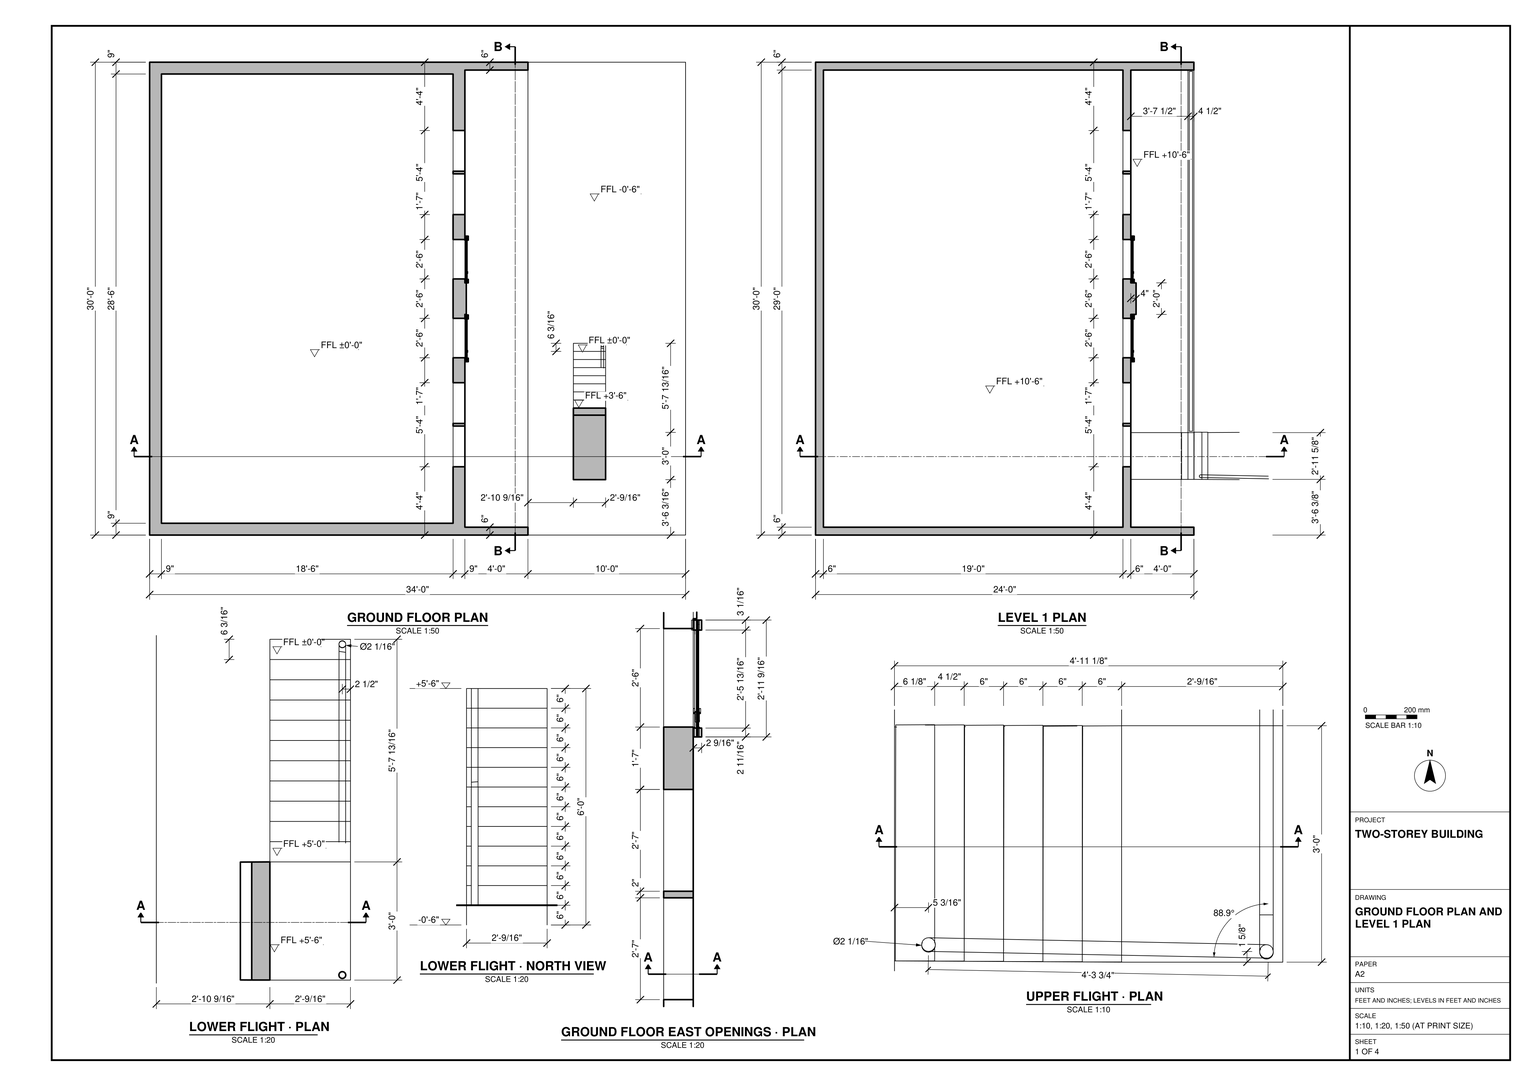
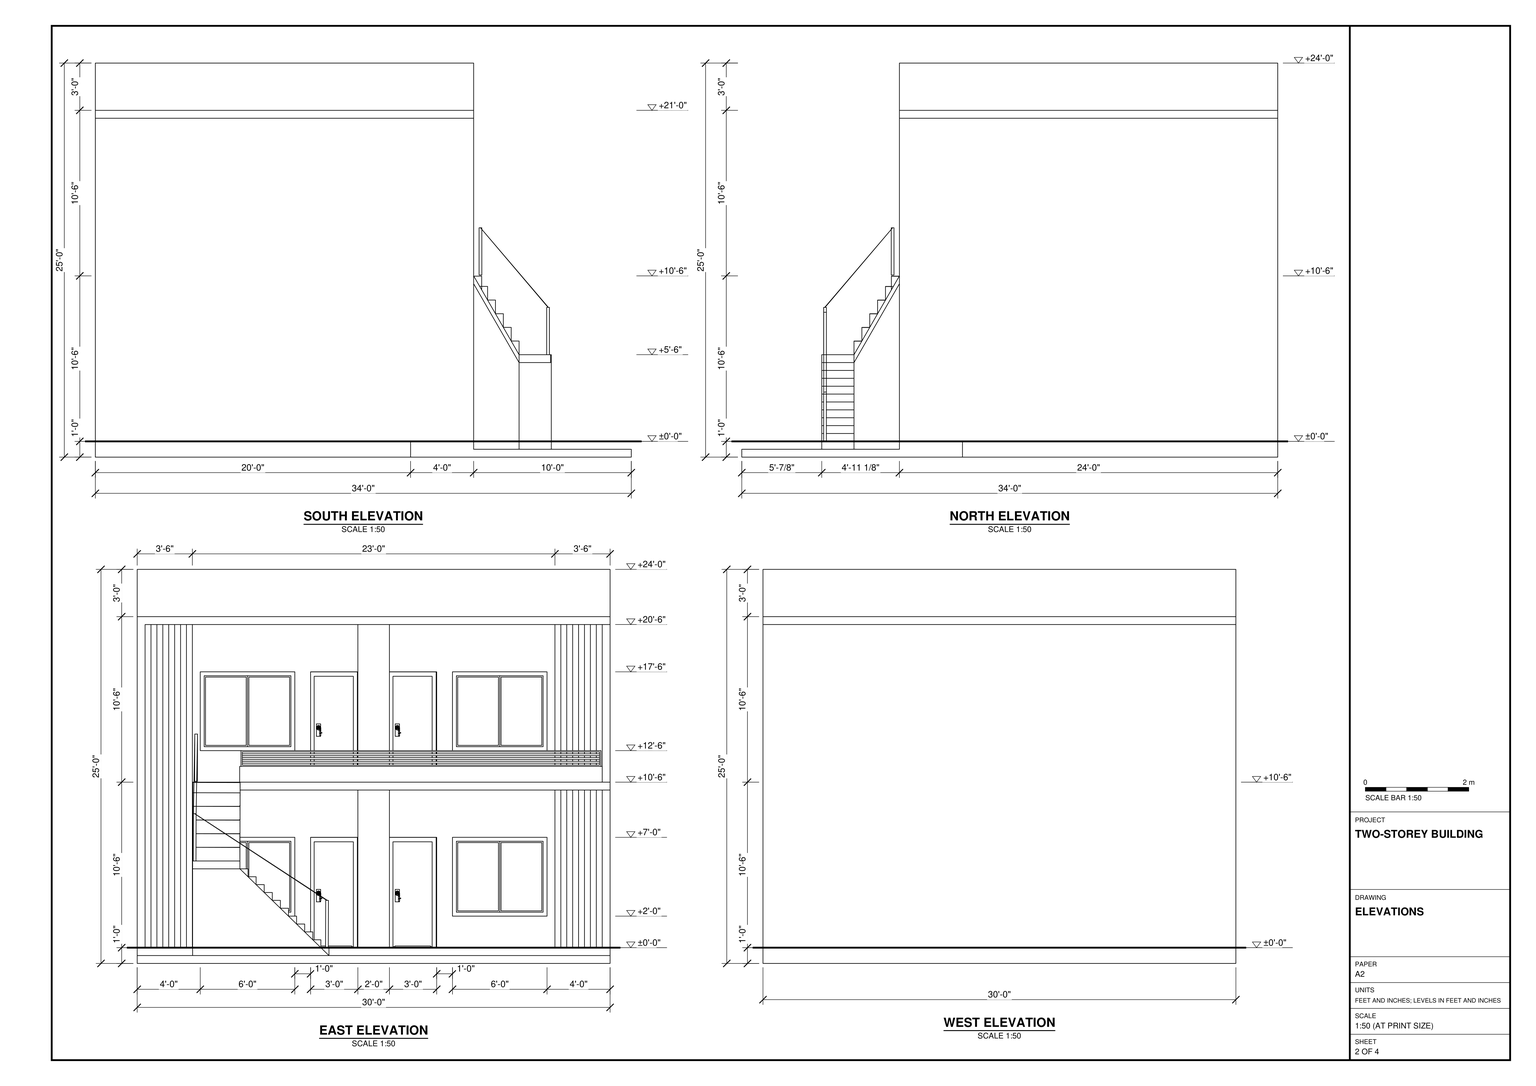
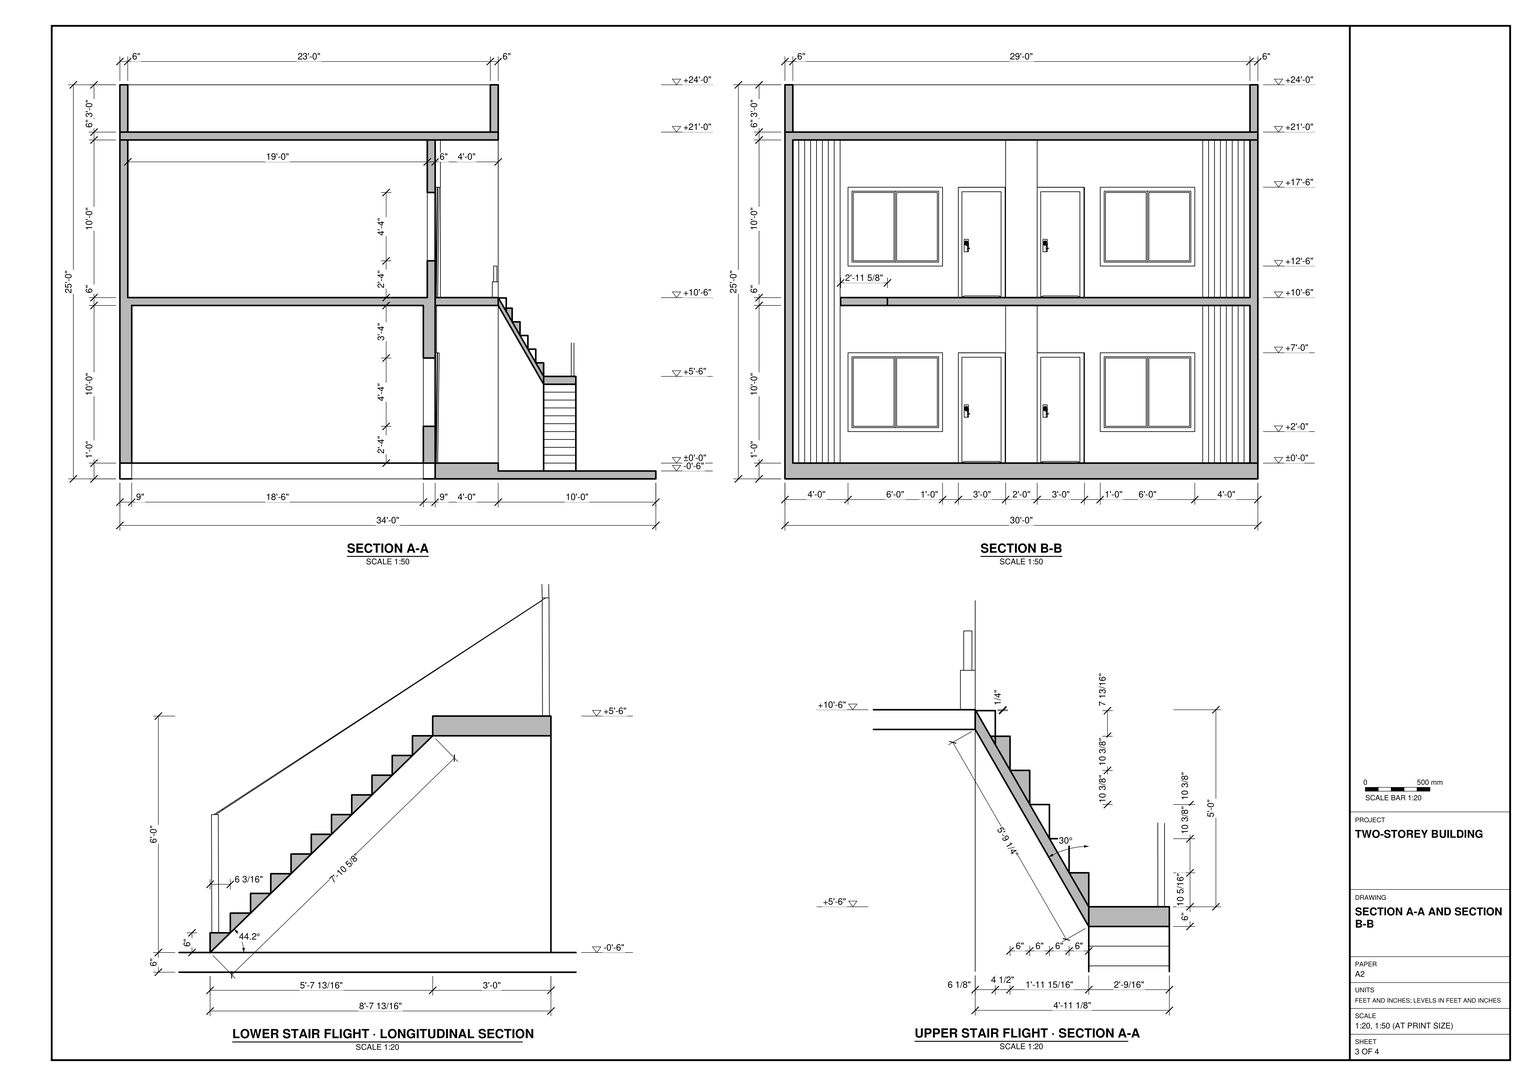
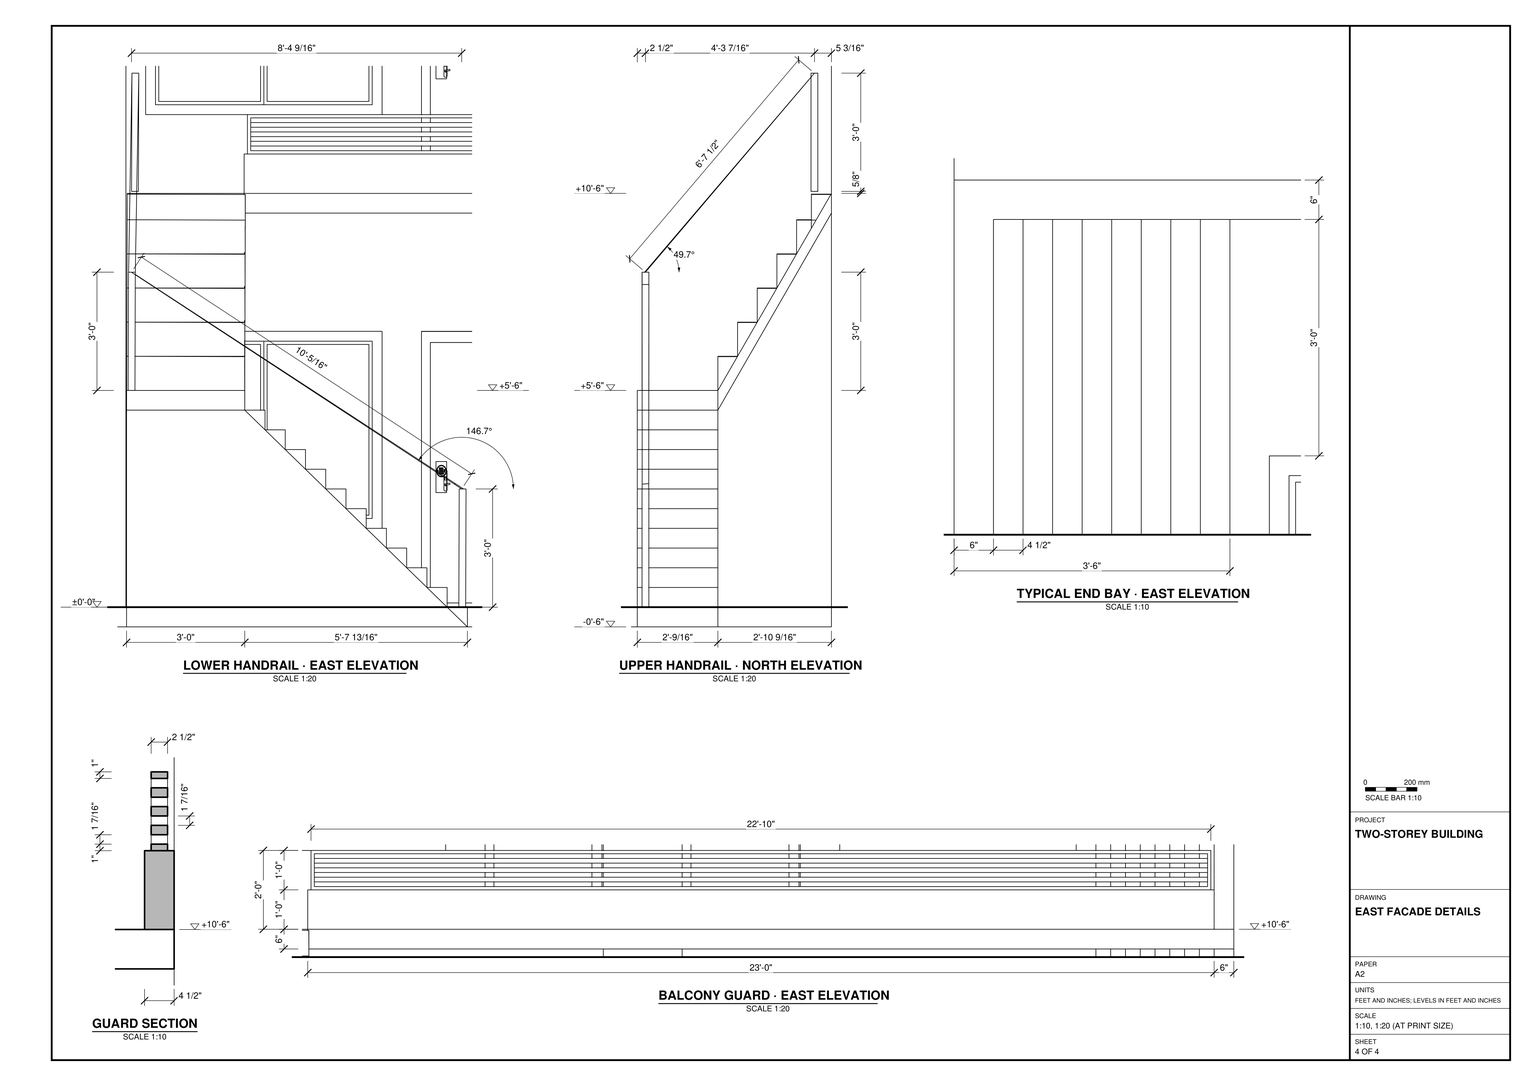
Build the two-storey building in SketchUp using task_files/diagram_01.pdf. Work in feet and inches. The overall model, including the base slab, is 34'-0" east to west, 30'-0" north to south and 25'-0" from the underside of the base to the top of the parapet. Set the ground floor at ±0'-0" and the upper floor at +10'-6".

Model the open rectangular room on each floor. Follow the plans for wall thicknesses, including the change from 9" around the ground-floor room to 6" around the upper room. On the east side, set the wall containing the doors and windows back from the ends of the side walls. On each floor, place two doors between a pair of framed windows, each with a central vertical division. Extend the upper slab along this frontage to form the access gallery and model its outer railing as shown in the east elevation.

Step the exterior base slab down on the east side. Build the lower stair flight parallel to the frontage, with individual treads rising to the landing at +5'-6". Turn the upper flight toward the building to meet the gallery, and include the stair handrails. Finish the shell with the flat roof slab and raised perimeter parapet shown in section.

Keep walls, slabs, roof and stair assemblies separately grouped, keep each furniture or joinery piece in its own group or component, and use components for repeated parts. Any decor or loose items shown may use suitable library components. Save one SketchUp model as output_files/two_storey_building_with_exterior_stair_and_gallery.skp.

# SketchUp Ruby script. Lengths in inches.
U = 1.inch
M = Sketchup.active_model
def pt(a) = Geom::Point3d.new(a.map { |v| v * U })
def face(e, loops, mat)
  f = e.add_face(loops[0].map { |a| pt(a) })
  loops[1..].each { |l| e.add_face(l.map { |a| pt(a) }).erase! }
  f.material = f.back_material = mat if mat
  f
end
# faces: each face lists its corners as indices into pts; further lists are holes
def faces(e, pts, list, mat = nil) = list.each { |f| face(e, (f[0].is_a?(Array) ? f : [f]).map { |l| l.map { |i| pts[i] } }, mat) }
# xy, xz, yz: faces in a plane at the given z, y or x. An outline is a flat list of corners, or four numbers for a rectangle; further outlines are holes
def ring(l) = l.size == 4 ? [[l[0], l[1]], [l[2], l[1]], [l[2], l[3]], [l[0], l[3]]] : l.each_slice(2).to_a
def flat(e, list, mat, &to3) = list.each { |f| face(e, (f[0].is_a?(Array) ? f : [f]).map { |l| ring(l).map { |u, v| to3.(u, v) } }, mat) }
def xy(e, z, list, mat = nil) = flat(e, list, mat) { |x, y| [x, y, z] }
def xz(e, y, list, mat = nil) = flat(e, list, mat) { |x, z| [x, y, z] }
def yz(e, x, list, mat = nil) = flat(e, list, mat) { |y, z| [x, y, z] }
def lines(e, pts, list) = list.each { |a, b| e.add_line(pt(pts[a]), pt(pts[b])) }
# prism: a flat outline (further loops are holes) pulled along v
def prism(e, loops, v, mat = nil)
  f = face(e, loops, mat); d = Geom::Vector3d.new(v.map { |x| x * U })
  f.pushpull(f.normal.samedirection?(d) ? d.length : -d.length)
end
def box(e, o, s, mat = nil) = prism(e, [[o, [o[0] + s[0], o[1], o[2]], [o[0] + s[0], o[1] + s[1], o[2]], [o[0], o[1] + s[1], o[2]]]], [0, 0, s[2]], mat)
def at(x, y, z, deg = 0) = Geom::Transformation.translation(pt([x, y, z])) * Geom::Transformation.rotation(ORIGIN, Z_AXIS, deg.degrees)
def axes(o, x, y, z) = Geom::Transformation.new([*x, 0, *y, 0, *z, 0, *pt(o).to_a, 1])
def part(name) = M.definitions.add(name)
# library, detail: a bought-in or finely detailed component or shape, given as its bounding box
def library(name, o, s) = part(name).tap { |d| box(d.entities, o, s) }
def detail(e, o, s) = box(e.add_group.entities, o, s)
def put(e, d, t, mat = nil) = e.add_instance(d, t).tap { |i| i.material = mat if mat }
def group(e, t, mat = nil) = e.add_group.tap { |g| g.transformation = t; g.material = mat if mat }.entities
root = M.entities
M.materials.add("Brick_05_1K").color = [195, 185, 161]
M.materials.add("Carpet_04_1K").color = [43, 65, 85]
M.materials.add("D01_Frost_White").color = [254, 255, 241]
M.materials.add("Glass_Basic_01").color = [136, 147, 158]
M.materials["Glass_Basic_01"].alpha = 0.6
M.materials.add("Plywood_01_1K").color = [125, 96, 64]
M.materials.add("Wood_Veneer_15_1K").color = [103, 69, 45]
M.materials.add("[Color_009]1").color = [0, 0, 0]
c1 = library("porta+4",[0.2,-5.42,1.33],[46.55,4.72,83.21])
c2 = part("Group\#3")
xy(c2.entities,6,[[0,0,24.54,6.16]])
xz(c2.entities,6.16,[[0,0,24.54,6]])
yz(c2.entities,0,[[6.16,0,0,6,6.16,6]])
yz(c2.entities,24.54,[[6.16,0,6.16,6,0,6]])
g1 = group(root,at(0,0,0),"D01_Frost_White")
xy(g1,0,[[[0,0,240,360],[9,9,231,351]]])
xy(g1,12,[[9,9,231,351]])
xz(g1,0,[[0,0,240,12]])
xz(g1,360,[[0,0,240,12]])
yz(g1,0,[[0,0,360,12]])
yz(g1,240,[[0,0,360,12]])
p = [[231,9,0],[231,9,12],[9,9,0],[9,9,12],[9,351,0],[9,351,12],
  [231,351,0],[231,351,12]]
lines(g1,p,[[0,1],[2,3],[4,5],[6,7]])
g2 = group(g1,at(0,0,12))
prism(g2,[[[294.08,44.24,126.62],[293.92,44.02,126.62],[293.7,43.86,126.62],[293.45,43.75,126.62],[293.18,43.72,126.62],[292.91,43.75,126.62],[292.66,43.86,126.62],[292.44,44.02,126.62],[292.28,44.24,126.62],[292.17,44.49,126.62],[292.14,44.76,126.62],[292.17,45.03,126.61],[292.28,45.28,126.61],[292.44,45.49,126.61],[292.66,45.66,126.61],[292.91,45.76,126.61],[293.18,45.8,126.61],[293.45,45.76,126.61],[293.7,45.66,126.61],[293.92,45.49,126.61],[294.08,45.28,126.61],[294.19,45.03,126.61],[294.22,44.76,126.62],[294.19,44.49,126.62]]],[0,0.12,36])
xy(g2,-12,[[240,0,408,360]])
xy(g2,-6,[[[288,0,408,360],[322.58,78.19,347.12,145.98]],[322.58,42.19,347.12,78.19],[322.58,78.19,347.12,145.98]])
xy(g2,0,[[[0,0,240,360],[9,9,231,351]],[240,6,288,6,288,354,240,354,240,192,241.07,192,241.07,168,240,168],[240,354,288,360]])
xy(g2,0,[[240,168,241.07,192]],"Brick_05_1K")
xy(g2,3,[[231,135,240,165],[231,195,240,225]])
xy(g2,28,[[231,52,240,83],[231,85,240,116],[231,244,240,275],[231,277,240,308]])
xy(g2,60,[[322.58,42.19,347.12,78.19]])
xy(g2,66,[[322.58,42.19,347.12,78.19],[344.63,42.66,344.37,42.7,344.11,42.8,343.9,42.97,343.73,43.18,343.63,43.43,343.59,43.7,343.63,43.97,343.73,44.22,343.9,44.44,344.11,44.61,344.37,44.71,344.63,44.74,344.9,44.71,345.15,44.61,345.37,44.44,345.54,44.22,345.64,43.97,345.68,43.7,345.64,43.43,345.54,43.18,345.37,42.97,345.15,42.8,344.9,42.7]])
xy(g2,80,[[231,52,240,83],[231,85,240,116],[231,244,240,275],[231,277,240,308]])
xy(g2,81,[[231,135,240,165],[231,195,240,225]])
xy(g2,102,[[344.63,42.78,344.9,42.8125,345.15,42.92,345.37,43.08,345.54,43.3,345.64,43.55,345.66,43.68,345.67,43.82,345.64,44.09,345.54,44.34,345.37,44.56,345.15,44.72,344.9,44.82,344.63,44.86,344.36,44.82,344.11,44.72,343.9,44.56,343.73,44.34,343.63,44.09,343.59,43.82,343.63,43.55,343.73,43.3,343.9,43.08,344.11,42.92,344.36,42.8125]])
xy(g2,120,[[9,9,231,351],[240,42.38,288,78],[240,78,240,168,241.07,168,241.07,192,240,192,240,354,288,354,288,78]])
xy(g2,120,[[240,168,241.07,180],[240,180,241.07,192]],"Brick_05_1K")
xy(g2,126,[[6,6,234,354],[240,42.38,278.67,78],[278.67,42.38,283.5,78],[283.5,42.38,288,78],[240,78,283.5,78,283.5,354,240,354,240,192,244,192,244,168,240,168],
  [283.5,78,288,354]])
xy(g2,126,[[240,168,244,180],[240,180,244,192]],"Brick_05_1K")
xy(g2,129,[[234,135,240,165],[234,195,240,225]])
xy(g2,138,[[284.5,79,287,353]])
xy(g2,138,[[[283.5,78,288,354],[284.5,79,287,353]]],"Carpet_04_1K")
xy(g2,139,[[284.5,80,287,352]],"[Color_009]1")
xy(g2,140.43,[[284.5,80,287,352]])
xy(g2,141.86,[[284.5,80,287,352]],"[Color_009]1")
xy(g2,143.29,[[284.5,80,287,352]])
xy(g2,144.71,[[284.5,80,287,352]],"[Color_009]1")
xy(g2,146.14,[[284.5,80,287,352]])
xy(g2,147.57,[[284.5,80,287,352]],"[Color_009]1")
xy(g2,149,[[284.5,80,287,352]])
xy(g2,150,[[284.5,79,287,353]],"[Color_009]1")
xy(g2,154,[[234,52,240,83],[234,85,240,116],[234,244,240,275],[234,277,240,308]])
xy(g2,206,[[234,52,240,83],[234,85,240,116],[234,244,240,275],[234,277,240,308]])
xy(g2,207,[[234,135,240,165],[234,195,240,225]])
xy(g2,246,[[0,0,6,354],[6,6,234,354],[234,6,234,354,240,354,240,192,244,192,244,168,240,168,240,6],[240,6,240,168,244,168,244,192,240,192,240,354,288,354,288,6],[0,354,288,360]])
xy(g2,252,[[[0,0,288,360],[6,6,282,354]],[6,6,282,354]])
xy(g2,288,[[[0,0,288,360],[6,6,282,354]]],"Carpet_04_1K")
xz(g2,0,[[240,-12,408,-12,408,-6,288,-6,288,246,0,246,0,0,240,0],[0,246,288,252]])
xz(g2,0,[[0,252,288,288]],"Carpet_04_1K")
xz(g2,6,[[240,0,288,246],[6,126,234,246]])
xz(g2,6,[[6,252,282,288]],"Carpet_04_1K")
xz(g2,9,[[9,0,231,120]])
xz(g2,42.19,[[322.58,-6,347.12,60],[322.58,60,346.58,66],[346.58,60,347.12,66]])
xz(g2,42.38,[[240,120,288,126]])
xz(g2,52,[[231,28,240,80],[234,154,240,206]])
xz(g2,78,[[240,120,288,126]])
xz(g2,78,[[283.5,126,288,138]],"Carpet_04_1K")
xz(g2,78.19,[[322.58,60,347.12,66]])
xz(g2,79,[[284.5,138,287,150]],"[Color_009]1")
xz(g2,80,[[284.5,139,287,140.43],[284.5,141.86,287,143.29],[284.5,144.71,287,146.14],[284.5,147.57,287,149]])
xz(g2,83,[[231,28,240,80],[234,154,240,206]])
xz(g2,85,[[231,28,240,80],[234,154,240,206]])
xz(g2,116,[[231,28,240,80],[234,154,240,206]])
xz(g2,135,[[231,3,240,81],[234,129,240,207]])
xz(g2,165,[[231,3,240,81],[234,129,240,207]])
xz(g2,168,[[240,0,241.07,84],[240,84,241.07,120],[240,126,244,210],[240,210,244,246]],"Brick_05_1K")
xz(g2,192,[[240,0,241.07,84],[240,84,241.07,120],[240,126,244,210],[240,210,244,246]],"Brick_05_1K")
xz(g2,195,[[231,3,240,81],[234,129,240,207]])
xz(g2,225,[[231,3,240,81],[234,129,240,207]])
xz(g2,244,[[231,28,240,80],[234,154,240,206]])
xz(g2,275,[[231,28,240,80],[234,154,240,206]])
xz(g2,277,[[231,28,240,80],[234,154,240,206]])
xz(g2,308,[[231,28,240,80],[234,154,240,206]])
xz(g2,351,[[9,0,231,120]])
xz(g2,352,[[284.5,139,287,140.43],[284.5,141.86,287,143.29],[284.5,144.71,287,146.14],[284.5,147.57,287,149]])
xz(g2,353,[[284.5,138,287,150]])
xz(g2,354,[[240,0,288,120],[6,126,234,246],[240,126,283.5,126,283.5,138,288,138,288,246,240,246],[283.5,126,288,138]])
xz(g2,354,[[6,252,282,288]],"Carpet_04_1K")
xz(g2,360,[[240,-12,240,0,288,0,288,-6,408,-6,408,-12],[0,0,288,246],[0,246,288,252]])
xz(g2,360,[[0,252,288,288]],"Carpet_04_1K")
yz(g2,0,[[0,0,360,246],[0,246,360,252]])
yz(g2,0,[[0,252,360,288]],"Carpet_04_1K")
yz(g2,6,[[6,126,354,246]])
yz(g2,6,[[6,252,354,288]],"Carpet_04_1K")
yz(g2,9,[[9,0,351,120]])
yz(g2,231,[[[9,0,351,120],[195,3,225,81],[135,3,165,81],[244,28,275,80],[277,28,308,80],[85,28,116,80],[52,28,83,80]]])
yz(g2,234,[[[6,126,354,246],[135,129,165,207],[195,129,225,207],[85,154,116,206],[244,154,275,206],[277,154,308,206],[52,154,83,206]]])
yz(g2,240,[[0,-12,360,0],[[42,0,132,0,132,84,168,84,168,120,42.38,120,42.38,126,132,126,132,210,168,210,168,246,42,246],[48,24,120,84],[48,150,120,210]],[[228,0,318,0,318,120,192,120,192,84,228,84],[240,24,312,84]],[42.38,120,78,126],[168,120,180,126],
  [180,120,192,126],[[228,126,318,126,318,246,192,246,192,210,228,210],[240,150,312,210]]])
yz(g2,240,[[52,28,83,80],[85,28,116,80],[244,28,275,80],[277,28,308,80],[52,154,83,206],
  [85,154,116,206],[244,154,275,206],[277,154,308,206]],"Glass_Basic_01")
yz(g2,240,[[6,0,10.5,246],[10.5,0,15,246],[15,0,19.5,246],[19.5,0,24,246],[24,0,28.5,246],
  [28.5,0,33,246],[33,0,37.5,246],[37.5,0,42,246],[318,0,322.5,120],[322.5,0,327,120],
  [327,0,331.5,120],[331.5,0,336,120],[336,0,340.5,120],[340.5,0,345,120],[345,0,349.5,120],
  [349.5,0,354,120],[[48,24,120,84],[51,27,117,81]],[[240,24,312,84],[243,27,309,81]],[[51,27,84,81],[52,28,83,80]],[[84,27,117,81],[85,28,116,80]],
  [[243,27,276,81],[244,28,275,80]],[[276,27,309,81],[277,28,308,80]],[318,126,322.5,246],[322.5,126,327,246],[327,126,331.5,246],
  [331.5,126,336,246],[336,126,340.5,246],[340.5,126,345,246],[345,126,349.5,246],[349.5,126,354,246],
  [[48,150,120,210],[51,153,117,207]],[[240,150,312,210],[243,153,309,207]],[[51,153,84,207],[52,154,83,206]],[[84,153,117,207],[85,154,116,206]],[[243,153,276,207],[244,154,275,206]],
  [[276,153,309,207],[277,154,308,206]]],"Plywood_01_1K")
yz(g2,240,[[[132,0,168,84],[135,3,165,81]],[[192,0,228,84],[195,3,225,81]],[[132,126,168,210],[135,129,165,207]],[[192,126,228,210],[195,129,225,207]]],"Wood_Veneer_15_1K")
yz(g2,241.07,[[168,0,192,120]],"Brick_05_1K")
yz(g2,244,[[168,126,192,246]],"Brick_05_1K")
yz(g2,282,[[6,252,354,288]],"Carpet_04_1K")
yz(g2,283.5,[[78,126,354,138]],"Carpet_04_1K")
yz(g2,284.5,[[[79,138,353,150],[80,147.57,352,149],[80,144.71,352,146.14],[80,141.86,352,143.29],[80,139,352,140.43]]],"[Color_009]1")
yz(g2,287,[[[79,138,353,150],[80,139,352,149]],[80,140.43,352,141.86],[80,143.29,352,144.71],[80,146.14,352,147.57]],"[Color_009]1")
yz(g2,288,[[0,-6,360,-6,360,0,6,0,6,246,360,246,360,252,0,252],[354,0,360,120],[42.38,120,78,126],[78,120,360,126],[354,126,360,246]])
yz(g2,288,[[78,126,354,138],[0,252,360,288]],"Carpet_04_1K")
yz(g2,294.12,[[42.35,115.39,78.35,115.39,78.35,125.67,42.38,125.78,42.36,117.98]])
yz(g2,298.61,[[42.33,107.59,78.33,107.59,78.33,117.87,42.36,117.98]])
yz(g2,304.6,[[42.29,97.19,78.29,97.19,78.29,107.47,42.33,107.59]])
yz(g2,310.6,[[42.26,86.79,78.26,86.79,78.26,97.08,42.29,97.19]])
yz(g2,316.59,[[42.23,76.4,78.23,76.4,78.23,86.68,42.26,86.79]])
yz(g2,322.58,[[42.19,-6,42.19,60,78.19,60,139.82,0,145.98,-6],[42.19,60,78.19,66],[42.19,66,78.19,66,78.19,76.28,42.23,76.4]])
yz(g2,347.12,[[42.19,-6,145.98,-6,139.82,0,78.19,60,42.19,60],[42.19,60,78.19,66]])
yz(g2,408,[[0,-12,360,-6]])
p = [[322.58,145.98,-6],[322.58,139.82,0],[347.12,139.82,0],[347.12,145.98,-6],[347.12,78.19,60],[322.58,78.19,60],
  [344.11,143.51,0],[344.37,143.4,0],[344.36,143.52,36],[344.11,143.625,36],[344.63,143.37,0],[344.63,143.48,36],
  [344.9,143.4,0],[344.9,143.52,36],[345.15,143.51,0],[345.15,143.625,36],[343.9,143.67,0],[343.9,143.79,36],
  [345.37,143.67,0],[345.37,143.79,36],[343.73,143.89,0],[343.73,144,36],[345.54,143.89,0],[345.54,144,36],
  [343.63,144.14,0],[343.63,144.26,36],[345.64,144.14,0],[345.64,144.26,36],[343.59,144.41,0],[343.59,144.53,36],
  [345.68,144.41,0],[345.67,144.53,36],[343.63,144.68,0],[343.63,144.79,36],[345.64,144.68,0],[345.64,144.79,36],
  [343.73,144.93,0],[343.73,145.05,36],[345.54,144.93,0],[345.54,145.05,36],[343.9,145.15,0],[343.9,145.26,36],
  [345.37,145.15,0],[345.37,145.26,36],[344.11,145.3125,0],[344.11,145.43,36],[345.15,145.3125,0],[345.15,145.43,36],
  [344.37,145.42,0],[344.36,145.53,36],[344.9,145.42,0],[344.9,145.53,36],[344.63,145.45,0],[344.63,145.57,36],
  [288,78,120],[322.58,42.19,60],[288,42.38,120],[322.58,42.19,66],[319.58,42.21,71.2],[316.59,42.23,76.4],
  [313.59,42.24,81.6],[310.6,42.26,86.79],[307.6,42.28,91.99],[304.6,42.29,97.19],[301.61,42.31,102.39],[298.61,42.33,107.59],
  [295.62,42.34,112.79],[294.12,42.35,115.39],[292.62,42.36,117.98],[291.12,42.37,120.58],[288.125,42.38,125.78],[288,42.38,126],
  [316.65,78.16,76.28],[322.58,78.19,66],[288,78,126],[288.19,78,125.67],[292.69,78.03,117.87],[294.12,78.03,115.39],
  [298.61,78.06,107.59],[298.68,78.06,107.47],[304.6,78.09,97.19],[304.67,78.09,97.08],[310.6,78.125,86.79],[310.66,78.125,86.68],
  [316.59,78.16,76.4],[322.58,42.23,76.4],[344.11,42.8,66],[344.37,42.7,66],[344.36,42.8125,102],[344.11,42.92,102],
  [344.63,42.66,66],[344.63,42.78,102],[344.9,42.7,66],[344.9,42.8125,102],[345.15,42.8,66],[345.15,42.92,102],
  [343.9,42.97,66],[343.9,43.08,102],[345.37,42.97,66],[345.37,43.08,102],[343.73,43.18,66],[343.73,43.3,102],
  [345.54,43.18,66],[345.54,43.3,102],[343.63,43.43,66],[343.63,43.55,102],[345.64,43.43,66],[345.64,43.55,102],
  [343.59,43.7,66],[343.59,43.82,102],[345.68,43.7,66],[345.67,43.82,102],[345.66,43.68,102],[343.63,43.97,66],
  [343.63,44.09,102],[345.64,43.97,66],[345.64,44.09,102],[343.73,44.22,66],[343.73,44.34,102],[345.54,44.22,66],
  [345.54,44.34,102],[343.9,44.44,66],[343.9,44.56,102],[345.37,44.44,66],[345.37,44.56,102],[344.11,44.61,66],
  [344.11,44.72,102],[345.15,44.61,66],[345.15,44.72,102],[344.37,44.71,66],[344.36,44.82,102],[344.9,44.71,66],
  [344.9,44.82,102],[344.63,44.74,66],[344.63,44.86,102],[322.58,78.19,76.28],[316.59,42.26,86.79],[310.66,78.19,86.68],
  [316.59,78.23,86.68],[316.59,78.23,76.4],[310.6,42.29,97.19],[304.67,78.23,97.08],[310.6,78.26,97.08],[310.6,78.26,86.79],
  [304.6,42.33,107.59],[298.68,78.26,107.47],[304.6,78.29,107.47],[304.6,78.29,97.19],[298.61,42.36,117.98],[294.12,42.36,117.98],
  [292.6875,78.29,117.87],[298.61,78.33,117.87],[298.61,78.33,107.59],[294.12,78.3,115.39],[288.19,78.32,125.67],[294.12,78.35,125.67],
  [294.12,78.35,115.39],[294.12,42.38,125.78],[9,9,120],[9,0,120],[9,351,120],[9,360,120],
  [231,351,120],[231,360,120],[293.18,43.83,162.62],[293.18,45.92,162.61],[345.64,142.01,37.47],[343.63,142.31,37.625],
  [345.66,49.39,98.25],[343.59,49.39,98.25]]
faces(g2,p,[[0,1,2,3],[4,2,1,5],[6,7,8,9],[7,10,11,8],[10,12,13,11],[12,14,15,13],[16,6,9,17],[14,18,19,15],
  [20,16,17,21],[18,22,23,19],[24,20,21,25],[22,26,27,23],[28,24,25,29],[26,30,31,27],[32,28,29,33],[30,34,35,31],
  [36,32,33,37],[34,38,39,35],[40,36,37,41],[38,42,43,39],[44,40,41,45],[42,46,47,43],[48,44,45,49],[46,50,51,47],
  [52,48,49,53],[50,52,53,51],[54,5,55,56],[57,58,59,60,61,62,63,64,65,66,67,68,69,70,71,56,55],[72,73,5,54,74,75,76,77,78,79,80,81,82,83,84],[57,85,59,58],[73,72,59,58,57],[86,87,88,89],
  [87,90,91,88],[90,92,93,91],[92,94,95,93],[96,86,89,97],[94,98,99,95],[100,96,97,101],[98,102,103,99],[104,100,101,105],
  [102,106,107,103],[108,104,105,109],[106,110,111,112,107],[113,108,109,114],[110,115,116,111],[117,113,114,118],[115,119,120,116],[121,117,118,122],
  [119,123,124,120],[125,121,122,126],[123,127,128,124],[129,125,126,130],[127,131,132,128],[133,129,130,134],[131,133,134,132],[72,135,73],
  [72,84,59],[85,135,72,59],[59,136,61,60],[84,83,61,60,59],[137,138,139],[136,138,137,83,61],[83,82,61],[61,140,63,62],
  [82,81,63,62,61],[141,142,143],[140,142,141,81,63],[81,80,63],[63,144,65,64],[80,79,65,64,63],[145,146,147],[144,146,145,79,65],
  [79,78,65],[148,149,67,66,65],[78,77,67,66,65],[150,151,152,153],[68,67,149],[68,67,77,76],[154,155,156],[76,75,70,69,68],
  [148,151,150,76,68,149],[69,68,149,157,70],[71,70,75,74],[157,155,154,75,70]])
lines(g2,p,[[158,159],[160,161],[162,163],[93,164],[165,134],[27,166],[33,167],[168,112],[168,169],[166,168],[167,109],[166,167]])
put(g2,c1,axes([237.64,131.85,-1.35],[0,0.76445,0],[-1,0,0],[0,0,1.0096]))
put(g2,c1,axes([237.64,191.85,-1.35],[0,0.76445,0],[-1,0,0],[0,0,1.0096]))
put(g2,c1,axes([237.64,131.85,124.65],[0,0.76445,0],[-1,0,0],[0,0,1.0096]))
put(g2,c1,axes([237.64,191.85,124.65],[0,0.76445,0],[-1,0,0],[0,0,1.0096]))
put(g2,c2,at(322.58,139.82,-6))
put(g2,c2,at(322.58,133.65,0))
put(g2,c2,at(322.58,127.49,6))
put(g2,c2,at(322.58,121.33,12))
put(g2,c2,at(322.58,115.17,18))
put(g2,c2,at(322.58,109,24))
put(g2,c2,at(322.58,102.84,30))
put(g2,c2,at(322.58,96.68,36))
put(g2,c2,at(322.58,90.52,42))
put(g2,c2,at(322.58,84.35,48))
put(g2,c2,at(322.58,78.19,54))
